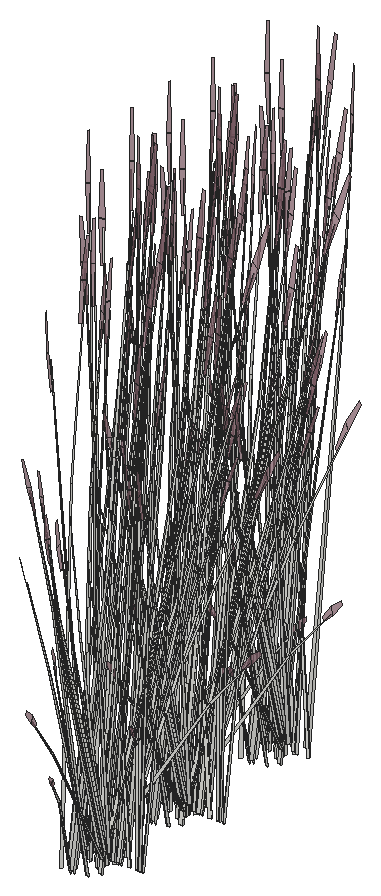
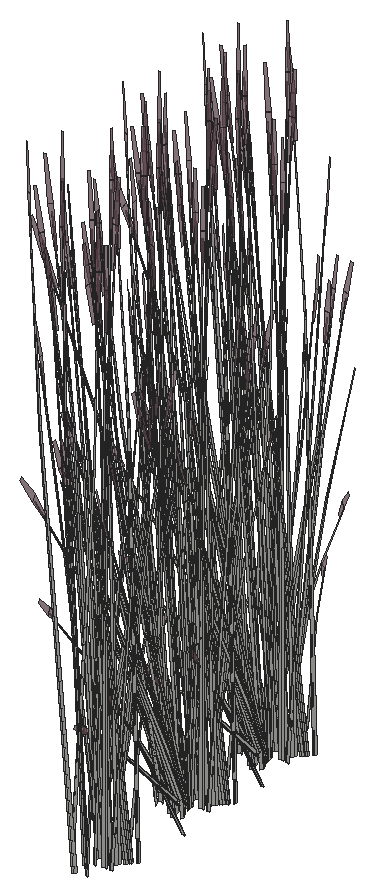
# SketchUp Ruby script. Lengths in inches.
U = 1.inch
M = Sketchup.active_model
def pt(a) = Geom::Point3d.new(a.map { |v| v * U })
def face(e, loops, mat)
  f = e.add_face(loops[0].map { |a| pt(a) })
  loops[1..].each { |l| e.add_face(l.map { |a| pt(a) }).erase! }
  f.material = f.back_material = mat if mat
  f
end
# faces: each face lists its corners as indices into pts; further lists are holes
def faces(e, pts, list, mat = nil) = list.each { |f| face(e, (f[0].is_a?(Array) ? f : [f]).map { |l| l.map { |i| pts[i] } }, mat) }
# xy, xz, yz: faces in a plane at the given z, y or x. An outline is a flat list of corners, or four numbers for a rectangle; further outlines are holes
def ring(l) = l.size == 4 ? [[l[0], l[1]], [l[2], l[1]], [l[2], l[3]], [l[0], l[3]]] : l.each_slice(2).to_a
def flat(e, list, mat, &to3) = list.each { |f| face(e, (f[0].is_a?(Array) ? f : [f]).map { |l| ring(l).map { |u, v| to3.(u, v) } }, mat) }
def xy(e, z, list, mat = nil) = flat(e, list, mat) { |x, y| [x, y, z] }
def xz(e, y, list, mat = nil) = flat(e, list, mat) { |x, z| [x, y, z] }
def yz(e, x, list, mat = nil) = flat(e, list, mat) { |y, z| [x, y, z] }
def lines(e, pts, list) = list.each { |a, b| e.add_line(pt(pts[a]), pt(pts[b])) }
# prism: a flat outline (further loops are holes) pulled along v
def prism(e, loops, v, mat = nil)
  f = face(e, loops, mat); d = Geom::Vector3d.new(v.map { |x| x * U })
  f.pushpull(f.normal.samedirection?(d) ? d.length : -d.length)
end
def box(e, o, s, mat = nil) = prism(e, [[o, [o[0] + s[0], o[1], o[2]], [o[0] + s[0], o[1] + s[1], o[2]], [o[0], o[1] + s[1], o[2]]]], [0, 0, s[2]], mat)
def at(x, y, z, deg = 0) = Geom::Transformation.translation(pt([x, y, z])) * Geom::Transformation.rotation(ORIGIN, Z_AXIS, deg.degrees)
def axes(o, x, y, z) = Geom::Transformation.new([*x, 0, *y, 0, *z, 0, *pt(o).to_a, 1])
def part(name) = M.definitions.add(name)
# library, detail: a bought-in or finely detailed component or shape, given as its bounding box
def library(name, o, s) = part(name).tap { |d| box(d.entities, o, s) }
def detail(e, o, s) = box(e.add_group.entities, o, s)
def put(e, d, t, mat = nil) = e.add_instance(d, t).tap { |i| i.material = mat if mat }
def group(e, t, mat = nil) = e.add_group.tap { |g| g.transformation = t; g.material = mat if mat }.entities
root = M.entities
M.materials.add("LightPink_Translucent").color = [144, 107, 117]
M.materials["LightPink_Translucent"].alpha = 0.75
c1 = part("blade")
p = [[2.15,0.21,22],[0,0.17,0],[0.09,0.45,0],[2.18,0.31,22],[2.29,0.31,22],[0.38,0.45,0],
  [2.48,0.24,33],[2.49,0.24,33],[2.48,0.22,33]]
faces(c1.entities,p,[[0,1,2,3],[4,5,2,3],[6,3,4,7],[8,0,3,6]])
c2 = part("seeds")
p = [[0.3,-0.1,1.38],[-0.01,-0.03,1.59],[-0.01,-0.03,0.03],[0.14,-0.07,-0.07],[0.29,-0.03,3],[0.15,0.01,3.11]]
faces(c2.entities,p,[[0,1,2,3],[1,0,4,5]],"LightPink_Translucent")
c3 = part("blade with seeds")
put(c3.entities,c1,at(0,0,0))
put(c3.entities,c2,axes([2.4,0.25,30.99],[1.5799,-0.05474,1.17369],[-0.12525,1.92788,0.29478],[-0.07173,-0.02425,1.56792]))
put(root,c3,axes([343.53,61.45,4.5],[0.43405,-0.58792,-0.44739],[0.90188,0.28295,0.21531],[0,-0.13553,1.43643]))
put(root,c3,axes([343.53,71.27,4.5],[0.43405,-0.58792,-0.44739],[0.90188,0.28295,0.21531],[0,-0.13553,1.43643]))
put(root,c3,axes([343.53,83.27,4.5],[0.43405,-0.58792,-0.44739],[0.90188,0.28295,0.21531],[0,-0.13553,1.43643]))
put(root,c3,axes([344.64,63.34,4.5],[-0.29189,-0.56252,0],[0.83351,-0.19699,0],[0,0,1.54371]))
put(root,c3,axes([344.64,73.17,4.5],[-0.29189,-0.56252,0],[0.83351,-0.19699,0],[0,0,1.54371]))
put(root,c3,axes([344.64,85.17,4.5],[-0.29189,-0.56252,0],[0.83351,-0.19699,0],[0,0,1.54371]))
put(root,c3,axes([343.58,64.53,3.79],[0.14478,-0.0355,1.76342],[0.8709,0.19542,-0.26939],[0.02547,0.22025,0.30037]))
put(root,c3,axes([343.58,74.36,3.79],[0.14478,-0.0355,1.76342],[0.8709,0.19542,-0.26939],[0.02547,0.22025,0.30037]))
put(root,c3,axes([343.77,64.73,6.82],[-0.2697,0.50175,-0.35414],[-0.78684,-0.14635,0.4572],[0.07215,0.20201,0.87481]))
put(root,c3,axes([343.77,74.55,6.82],[-0.2697,0.50175,-0.35414],[-0.78684,-0.14635,0.4572],[0.07215,0.20201,0.87481]))
put(root,c3,axes([345.81,62.23,4.5],[-0.43405,0.58792,-0.44739],[-0.90188,-0.28295,0.21531],[0,0.13553,1.43643]))
put(root,c3,axes([345.81,72.06,4.5],[-0.43405,0.58792,-0.44739],[-0.90188,-0.28295,0.21531],[0,0.13553,1.43643]))
put(root,c3,axes([345.35,58.9,7.02],[0.6592,-0.22175,0.0643],[0.32265,0.40436,0.50621],[-0.06366,-0.17825,0.77189]))
put(root,c3,axes([345.35,68.73,7.02],[0.6592,-0.22175,0.0643],[0.32265,0.40436,0.50621],[-0.06366,-0.17825,0.77189]))
put(root,c3,axes([345.35,80.73,7.02],[0.6592,-0.22175,0.0643],[0.32265,0.40436,0.50621],[-0.06366,-0.17825,0.77189]))
put(root,c3,axes([343.21,65.62,7.01],[0.1134,0.10507,1.74944],[0.91515,0.04128,-0.27667],[0.09203,0.23172,0.14031]))
put(root,c3,axes([343.21,75.44,7.01],[0.1134,0.10507,1.74944],[0.91515,0.04128,-0.27667],[0.09203,0.23172,0.14031]))
put(root,c3,axes([347.53,61.875,4.77],[-0.70288,-0.47526,0.17642],[0.70832,-0.46097,0.35086],[-0.07763,0.09706,1.60407]))
put(root,c3,axes([347.53,71.7,4.77],[-0.70288,-0.47526,0.17642],[0.70832,-0.46097,0.35086],[-0.07763,0.09706,1.60407]))
put(root,c3,axes([347.53,83.7,4.77],[-0.70288,-0.47526,0.17642],[0.70832,-0.46097,0.35086],[-0.07763,0.09706,1.60407]))
put(root,c3,axes([345.1,61.6,4.5],[0,-0.75495,0],[1.11865,0,0],[0,0,1.79456]))
put(root,c3,axes([345.1,71.43,4.5],[0,-0.75495,0],[1.11865,0,0],[0,0,1.79456]))
put(root,c3,axes([345.1,83.43,4.5],[0,-0.75495,0],[1.11865,0,0],[0,0,1.79456]))
put(root,c3,axes([345.12,58.95,7.03],[0.88151,0.17057,0.48003],[-0.30143,0.56078,0.3958],[-0.05297,-0.22053,0.9933]))
put(root,c3,axes([345.12,68.77,7.03],[0.88151,0.17057,0.48003],[-0.30143,0.56078,0.3958],[-0.05297,-0.22053,0.9933]))
put(root,c3,axes([345.12,80.77,7.03],[0.88151,0.17057,0.48003],[-0.30143,0.56078,0.3958],[-0.05297,-0.22053,0.9933]))
put(root,c3,axes([344.0625,61.74,4.73],[1.00799,0.31623,0.24065],[-0.48511,0.65709,0.50002],[0,-0.15147,1.60543]))
put(root,c3,axes([344.0625,71.57,4.73],[1.00799,0.31623,0.24065],[-0.48511,0.65709,0.50002],[0,-0.15147,1.60543]))
put(root,c3,axes([344.0625,83.57,4.73],[1.00799,0.31623,0.24065],[-0.48511,0.65709,0.50002],[0,-0.15147,1.60543]))
put(root,c3,axes([345.67,61.9,4.59],[0,0.75458,-0.05637],[-1.11865,0,0],[0,0.02371,1.79368]))
put(root,c3,axes([345.67,71.73,4.59],[0,0.75458,-0.05637],[-1.11865,0,0],[0,0.02371,1.79368]))
put(root,c3,axes([343.74,61.3,5.01],[-0.97146,0.04028,0.44739],[-0.08785,-0.66859,-0.21531],[0.17391,-0.06776,1.43643]))
put(root,c3,axes([343.74,71.125,5.01],[-0.97146,0.04028,0.44739],[-0.08785,-0.66859,-0.21531],[0.17391,-0.06776,1.43643]))
put(root,c3,axes([343.74,83.125,5.01],[-0.97146,0.04028,0.44739],[-0.08785,-0.66859,-0.21531],[0.17391,-0.06776,1.43643]))
put(root,c3,axes([343.68,64.2,7.34],[0.2697,-0.50175,0.35414],[0.78684,0.14635,-0.4572],[0.07215,0.20201,0.87481]))
put(root,c3,axes([343.68,74.03,7.34],[0.2697,-0.50175,0.35414],[0.78684,0.14635,-0.4572],[0.07215,0.20201,0.87481]))
put(root,c3,axes([343.29,60.15,4.77],[-0.25843,0.64844,0.17642],[-0.9457,-0.1835,0.35086],[0.16336,-0.00316,1.60407]))
put(root,c3,axes([343.29,69.98,4.77],[-0.25843,0.64844,0.17642],[-0.9457,-0.1835,0.35086],[0.16336,-0.00316,1.60407]))
put(root,c3,axes([343.29,81.98,4.77],[-0.25843,0.64844,0.17642],[-0.9457,-0.1835,0.35086],[0.16336,-0.00316,1.60407]))
put(root,c3,axes([345.13,63.36,4.58],[0.38895,0.74956,-0.06012],[-1.11135,0.26265,0],[0.01358,0.02618,1.72173]))
put(root,c3,axes([345.13,73.1875,4.58],[0.38895,0.74956,-0.06012],[-1.11135,0.26265,0],[0.01358,0.02618,1.72173]))
put(root,c3,axes([342.82,59.35,4.67],[-0.55932,-0.6538,0],[0.93577,-0.36461,-0.51607],[0.21313,-0.08304,1.63711]))
put(root,c3,axes([342.82,69.18,4.67],[-0.55932,-0.6538,0],[0.93577,-0.36461,-0.51607],[0.21313,-0.08304,1.63711]))
put(root,c3,axes([342.82,81.18,4.67],[-0.55932,-0.6538,0],[0.93577,-0.36461,-0.51607],[0.21313,-0.08304,1.63711]))
put(root,c3,axes([343.85,64.28,7.27],[0.42698,0.53052,-0.71045],[-0.87893,0.29566,0.08574],[0.09984,0.25633,1.00501]))
put(root,c3,axes([343.85,74.1,7.27],[0.42698,0.53052,-0.71045],[-0.87893,0.29566,0.08574],[0.09984,0.25633,1.00501]))
put(root,c3,axes([348.34,62.38,4.49],[-1.1181,-0.00522,-0.04976],[0,-0.72922,0.49943],[-0.03514,0.166,1.58352]))
put(root,c3,axes([348.34,72.21,4.49],[-1.1181,-0.00522,-0.04976],[0,-0.72922,0.49943],[-0.03514,0.166,1.58352]))
put(root,c3,axes([346.15,60.1875,4.77],[-0.96132,0.17317,0.17642],[-0.23737,-0.64447,0.35086],[0.08574,0.0939,1.60407]))
put(root,c3,axes([346.15,70.01,4.77],[-0.96132,0.17317,0.17642],[-0.23737,-0.64447,0.35086],[0.08574,0.0939,1.60407]))
put(root,c3,axes([346.15,82.01,4.77],[-0.96132,0.17317,0.17642],[-0.23737,-0.64447,0.35086],[0.08574,0.0939,1.60407]))
put(root,c3,axes([345.16,57.77,5.06],[0.11476,0.38047,1.1486],[-0.63664,-0.21072,0.84392],[0.06851,-0.19481,0.25299]))
put(root,c3,axes([345.16,67.6,5.06],[0.11476,0.38047,1.1486],[-0.63664,-0.21072,0.84392],[0.06851,-0.19481,0.25299]))
put(root,c3,axes([345.16,79.6,5.06],[0.11476,0.38047,1.1486],[-0.63664,-0.21072,0.84392],[0.06851,-0.19481,0.25299]))
put(root,c3,axes([344.74,65.99,7.9375],[0.61821,-0.37431,-0.06488],[0.56645,0.40995,-0.29416],[0.03988,0.11616,0.97024]))
put(root,c3,axes([344.74,75.82,7.9375],[0.61821,-0.37431,-0.06488],[0.56645,0.40995,-0.29416],[0.03988,0.11616,0.97024]))
put(root,c3,axes([344.57,61.125,4.65],[-0.74176,0.59212,0.45755],[-0.88124,-0.52269,0.17955],[0.17882,-0.05909,1.58856]))
put(root,c3,axes([344.57,70.95,4.65],[-0.74176,0.59212,0.45755],[-0.88124,-0.52269,0.17955],[0.17882,-0.05909,1.58856]))
put(root,c3,axes([344.57,82.95,4.65],[-0.74176,0.59212,0.45755],[-0.88124,-0.52269,0.17955],[0.17882,-0.05909,1.58856]))
put(root,c3,axes([345.84,62.06,4.51],[0.62448,0.42144,0],[-0.62448,0.42144,0],[0,0,1.69266]))
put(root,c3,axes([345.84,71.89,4.51],[0.62448,0.42144,0],[-0.62448,0.42144,0],[0,0,1.69266]))
put(root,c3,axes([345.84,83.89,4.51],[0.62448,0.42144,0],[-0.62448,0.42144,0],[0,0,1.69266]))
put(root,c3,axes([345.83,61.57,5.01],[0.43405,-0.58792,0.44739],[0.90188,0.28295,-0.21531],[0,0.13553,1.43643]))
put(root,c3,axes([345.83,71.39,5.01],[0.43405,-0.58792,0.44739],[0.90188,0.28295,-0.21531],[0,0.13553,1.43643]))
put(root,c3,axes([345.83,83.39,5.01],[0.43405,-0.58792,0.44739],[0.90188,0.28295,-0.21531],[0,0.13553,1.43643]))
put(root,c3,axes([345.45,63.61,4.5],[0.90188,0.29293,0],[-0.43405,0.60866,0],[0,0,1.74954]))
put(root,c3,axes([345.45,73.44,4.5],[0.90188,0.29293,0],[-0.43405,0.60866,0],[0,0,1.74954]))
put(root,c3,axes([344.17,64.38,6.97],[0.87941,0.16356,-0.51099],[-0.30143,0.56078,-0.3958],[0.08064,0.22578,0.97773]))
put(root,c3,axes([344.17,74.21,6.97],[0.87941,0.16356,-0.51099],[-0.30143,0.56078,-0.3958],[0.08064,0.22578,0.97773]))
put(root,c3,axes([343.42,64.41,7.33],[0.87543,-0.30377,-0.1216],[0.4302,0.53915,-0.67495],[0.1155,0.2272,1.02557]))
put(root,c3,axes([343.42,74.24,7.33],[0.87543,-0.30377,-0.1216],[0.4302,0.53915,-0.67495],[0.1155,0.2272,1.02557]))
put(root,c3,axes([345.54,61.43,4.67],[-1.13071,-0.13747,0.49198],[0.23011,-0.77639,0.19306],[0.16524,0.07497,1.70813]))
put(root,c3,axes([345.54,71.25,4.67],[-1.13071,-0.13747,0.49198],[0.23011,-0.77639,0.19306],[0.16524,0.07497,1.70813]))
put(root,c3,axes([345.54,83.25,4.67],[-1.13071,-0.13747,0.49198],[0.23011,-0.77639,0.19306],[0.16524,0.07497,1.70813]))
put(root,c3,axes([347.89,58.39,7],[-0.09085,0.04984,1.77383],[-0.89014,-0.16814,-0.16761],[-0.03222,-0.21748,0.31391]))
put(root,c3,axes([347.89,68.22,7],[-0.09085,0.04984,1.77383],[-0.89014,-0.16814,-0.16761],[-0.03222,-0.21748,0.31391]))
put(root,c3,axes([347.89,80.22,7],[-0.09085,0.04984,1.77383],[-0.89014,-0.16814,-0.16761],[-0.03222,-0.21748,0.31391]))
put(root,c3,axes([347.19,59.83,7.33],[-0.98321,-0.03233,-0.1216],[0.02687,-0.61208,-0.67495],[0.0683,-0.23574,1.02557]))
put(root,c3,axes([347.19,69.66,7.33],[-0.98321,-0.03233,-0.1216],[0.02687,-0.61208,-0.67495],[0.0683,-0.23574,1.02557]))
put(root,c3,axes([347.19,81.66,7.33],[-0.98321,-0.03233,-0.1216],[0.02687,-0.61208,-0.67495],[0.0683,-0.23574,1.02557]))
put(root,c3,axes([348.11,62.49,4.32],[-0.62448,0.40708,-0.30978],[-0.62448,-0.40708,0.30978],[0,0.13112,1.38974]))
put(root,c3,axes([348.11,72.3125,4.32],[-0.62448,0.40708,-0.30978],[-0.62448,-0.40708,0.30978],[0,0.13112,1.38974]))
put(root,c3,axes([346.33,62.41,4.39],[0.32803,0.59738,-0.69212],[-0.94492,0.21515,-0.18165],[0.03626,0.20229,1.52773]))
put(root,c3,axes([346.33,72.24,4.39],[0.32803,0.59738,-0.69212],[-0.94492,0.21515,-0.18165],[0.03626,0.20229,1.52773]))
put(root,c3,axes([345.86,61.77,4.5],[1.00089,0,0],[0,0.67548,0],[0,0,1.78407]))
put(root,c3,axes([345.86,71.6,4.5],[1.00089,0,0],[0,0.67548,0],[0,0,1.78407]))
put(root,c3,axes([345.86,83.6,4.5],[1.00089,0,0],[0,0.67548,0],[0,0,1.78407]))
put(root,c3,axes([346.81,59.92,7.34],[-0.60531,0.34352,0.35414],[-0.573,-0.39225,-0.4572],[0.08718,-0.19929,0.87481]))
put(root,c3,axes([346.81,69.75,7.34],[-0.60531,0.34352,0.35414],[-0.573,-0.39225,-0.4572],[0.08718,-0.19929,0.87481]))
put(root,c3,axes([346.81,81.75,7.34],[-0.60531,0.34352,0.35414],[-0.573,-0.39225,-0.4572],[0.08718,-0.19929,0.87481]))
put(root,c3,axes([344.9,61.02,5.01],[-0.53742,-0.54764,0.44739],[0.81403,-0.38564,-0.21531],[0.17391,0.06776,1.43643]))
put(root,c3,axes([344.9,70.85,5.01],[-0.53742,-0.54764,0.44739],[0.81403,-0.38564,-0.21531],[0.17391,0.06776,1.43643]))
put(root,c3,axes([344.9,82.85,5.01],[-0.53742,-0.54764,0.44739],[0.81403,-0.38564,-0.21531],[0.17391,0.06776,1.43643]))
put(root,c3,axes([343.92,61.16,4.96],[-0.10425,-0.7445,-0.29095],[1.08575,-0.04502,-0.50002],[0.19119,-0.09917,1.59708]))
put(root,c3,axes([343.92,70.98,4.96],[-0.10425,-0.7445,-0.29095],[1.08575,-0.04502,-0.50002],[0.19119,-0.09917,1.59708]))
put(root,c3,axes([343.92,82.98,4.96],[-0.10425,-0.7445,-0.29095],[1.08575,-0.04502,-0.50002],[0.19119,-0.09917,1.59708]))
put(root,c3,axes([346.21,61.7,4.91],[0.83351,-0.19028,0.1448],[0.29189,0.54335,-0.41347],[0,0.11958,1.26744]))
put(root,c3,axes([346.21,71.53,4.91],[0.83351,-0.19028,0.1448],[0.29189,0.54335,-0.41347],[0,0.11958,1.26744]))
put(root,c3,axes([346.52,59.6,6.97],[-0.64041,-0.4384,-0.51099],[0.67652,-0.38394,-0.3958],[0.09744,-0.22274,0.97773]))
put(root,c3,axes([346.52,69.43,6.97],[-0.64041,-0.4384,-0.51099],[0.67652,-0.38394,-0.3958],[0.09744,-0.22274,0.97773]))
put(root,c3,axes([346.52,81.43,6.97],[-0.64041,-0.4384,-0.51099],[0.67652,-0.38394,-0.3958],[0.09744,-0.22274,0.97773]))
put(root,c3,axes([345.92,61.74,4.96],[1.00749,0.31132,-0.29095],[-0.48511,0.65709,-0.50002],[0.03166,0.16133,1.59708]))
put(root,c3,axes([345.92,71.57,4.96],[1.00749,0.31132,-0.29095],[-0.48511,0.65709,-0.50002],[0.03166,0.16133,1.59708]))
put(root,c3,axes([343.78,59.51,4.32],[0.83462,0.16144,-0.30978],[-0.21015,0.56852,0.30978],[0.16826,-0.06556,1.38974]))
put(root,c3,axes([343.78,69.33,4.32],[0.83462,0.16144,-0.30978],[-0.21015,0.56852,0.30978],[0.16826,-0.06556,1.38974]))
put(root,c3,axes([343.78,81.33,4.32],[0.83462,0.16144,-0.30978],[-0.21015,0.56852,0.30978],[0.16826,-0.06556,1.38974]))
put(root,c3,axes([346.1,58.82,4.88],[-0.25429,0.13207,1.43002],[-0.76157,-0.23115,-0.30754],[0.14117,-0.28747,0.61141]))
put(root,c3,axes([346.1,68.65,4.88],[-0.25429,0.13207,1.43002],[-0.76157,-0.23115,-0.30754],[0.14117,-0.28747,0.61141]))
put(root,c3,axes([346.1,80.65,4.88],[-0.25429,0.13207,1.43002],[-0.76157,-0.23115,-0.30754],[0.14117,-0.28747,0.61141]))
put(root,c3,axes([348.11,61.89,4.77],[0,-0.65246,0.49651],[1.00089,0,0],[0,0.1486,1.57504]))
put(root,c3,axes([348.11,71.72,4.77],[0,-0.65246,0.49651],[1.00089,0,0],[0,0.1486,1.57504]))
put(root,c3,axes([348.54,62.5,4.3125],[0,0.65246,-0.49651],[-1.00089,0,0],[0,0.1486,1.57504]))
put(root,c3,axes([348.54,72.33,4.3125],[0,0.65246,-0.49651],[-1.00089,0,0],[0,0.1486,1.57504]))
put(root,c3,axes([345.87,64.48,7.03],[-0.88979,0.14973,0.48003],[-0.15442,-0.58737,0.3958],[0.20926,0.17311,0.9933]))
put(root,c3,axes([345.87,74.3,7.03],[-0.88979,0.14973,0.48003],[-0.15442,-0.58737,0.3958],[0.20926,0.17311,0.9933]))
put(root,c3,axes([343.58,59.25,4.3125],[0.83726,-0.32623,-0.49651],[0.50045,0.58498,0],[0.19069,-0.0743,1.57504]))
put(root,c3,axes([343.58,69.08,4.3125],[0.83726,-0.32623,-0.49651],[0.50045,0.58498,0],[0.19069,-0.0743,1.57504]))
put(root,c3,axes([343.58,81.08,4.3125],[0.83726,-0.32623,-0.49651],[0.50045,0.58498,0],[0.19069,-0.0743,1.57504]))
put(root,c3,axes([345.7,64.59,7.02],[-0.4066,0.41448,0.0643],[-0.57901,-0.24131,0.50621],[0.18719,0.13288,0.77189]))
put(root,c3,axes([345.7,74.42,7.02],[-0.4066,0.41448,0.0643],[-0.57901,-0.24131,0.50621],[0.18719,0.13288,0.77189]))
put(root,c3,axes([344.67,63.23,6.17],[-0.2045,-0.20949,1.71376],[0.94495,-0.17636,0.13857],[0.21357,0.32887,0.73262]))
put(root,c3,axes([344.67,73.05,6.17],[-0.2045,-0.20949,1.71376],[0.94495,-0.17636,0.13857],[0.21357,0.32887,0.73262]))
put(root,c3,axes([345.26,60.87,4.91],[0.17258,-0.58229,0.1448],[0.84319,0.10108,-0.41347],[0.15345,0.05979,1.26744]))
put(root,c3,axes([345.26,70.7,4.91],[0.17258,-0.58229,0.1448],[0.84319,0.10108,-0.41347],[0.15345,0.05979,1.26744]))
put(root,c3,axes([345.26,82.7,4.91],[0.17258,-0.58229,0.1448],[0.84319,0.10108,-0.41347],[0.15345,0.05979,1.26744]))
put(root,c3,axes([346.46,59.86,4.77],[-0.83726,-0.32623,0.49651],[0.50045,-0.58498,0],[0.19069,0.0743,1.57504]))
put(root,c3,axes([346.46,69.68,4.77],[-0.83726,-0.32623,0.49651],[0.50045,-0.58498,0],[0.19069,0.0743,1.57504]))
put(root,c3,axes([346.46,81.68,4.77],[-0.83726,-0.32623,0.49651],[0.50045,-0.58498,0],[0.19069,0.0743,1.57504]))
put(root,c3,axes([346.72,59.8,7.27],[0.02328,-0.60353,-0.71045],[0.98022,0.04053,0.08574],[0.10344,-0.25568,1.00501]))
put(root,c3,axes([346.72,69.625,7.27],[0.02328,-0.60353,-0.71045],[0.98022,0.04053,0.08574],[0.10344,-0.25568,1.00501]))
put(root,c3,axes([346.72,81.625,7.27],[0.02328,-0.60353,-0.71045],[0.98022,0.04053,0.08574],[0.10344,-0.25568,1.00501]))
put(root,c3,axes([345.73,63.26,4.48],[0.93921,-0.22138,-0.19198],[0.33003,0.6377,0.00008],[0.10367,-0.02447,1.73897]))
put(root,c3,axes([345.73,73.09,4.48],[0.93921,-0.22138,-0.19198],[0.33003,0.6377,0.00008],[0.10367,-0.02447,1.73897]))
put(root,c3,axes([345.73,85.09,4.48],[0.93921,-0.22138,-0.19198],[0.33003,0.6377,0.00008],[0.10367,-0.02447,1.73897]))
put(root,c3,axes([345.57,64.12,7.34],[-0.13817,-0.52554,0.35414],[0.78985,-0.13877,-0.4572],[0.21215,0.1506,0.87481]))
put(root,c3,axes([345.57,73.94,7.34],[-0.13817,-0.52554,0.35414],[0.78985,-0.13877,-0.4572],[0.21215,0.1506,0.87481]))
put(root,c3,axes([345.75,61.37,4.5],[0.53742,0.54764,-0.44739],[-0.81403,0.38564,0.21531],[0.17391,0.06776,1.43643]))
put(root,c3,axes([345.75,71.19,4.5],[0.53742,0.54764,-0.44739],[-0.81403,0.38564,0.21531],[0.17391,0.06776,1.43643]))
put(root,c3,axes([346.1,61.09,6.77],[-0.77304,-0.33901,1.38283],[0.81626,-0.52782,0.59665],[0.24941,0.31809,1.33663]))
put(root,c3,axes([346.1,70.92,6.77],[-0.77304,-0.33901,1.38283],[0.81626,-0.52782,0.59665],[0.24941,0.31809,1.33663]))
put(root,c3,axes([347.12,59.4375,6.82],[0.60531,-0.34352,-0.35414],[0.573,0.39225,0.4572],[0.08718,-0.19929,0.87481]))
put(root,c3,axes([347.12,69.26,6.82],[0.60531,-0.34352,-0.35414],[0.573,0.39225,0.4572],[0.08718,-0.19929,0.87481]))
put(root,c3,axes([347.12,81.26,6.82],[0.60531,-0.34352,-0.35414],[0.573,0.39225,0.4572],[0.08718,-0.19929,0.87481]))
put(root,c3,axes([344.8,64.85,7],[0.00265,-0.07899,1.77383],[0.76665,-0.34851,-0.16761],[0.2663,0.12439,0.31391]))
put(root,c3,axes([344.8,74.68,7],[0.00265,-0.07899,1.77383],[0.76665,-0.34851,-0.16761],[0.2663,0.12439,0.31391]))
